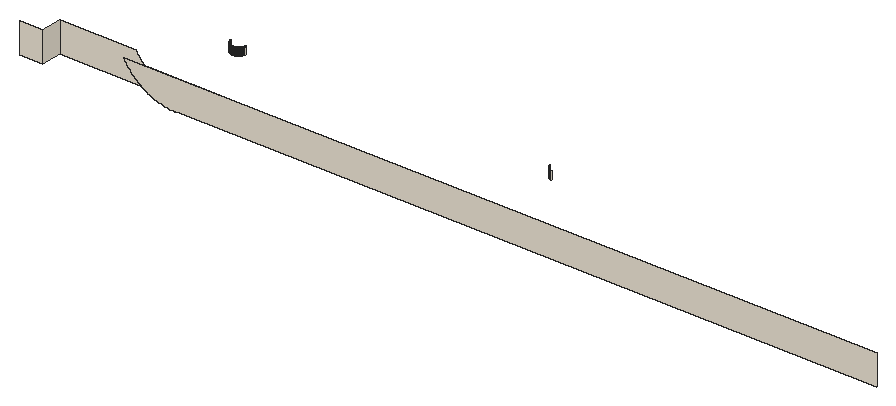
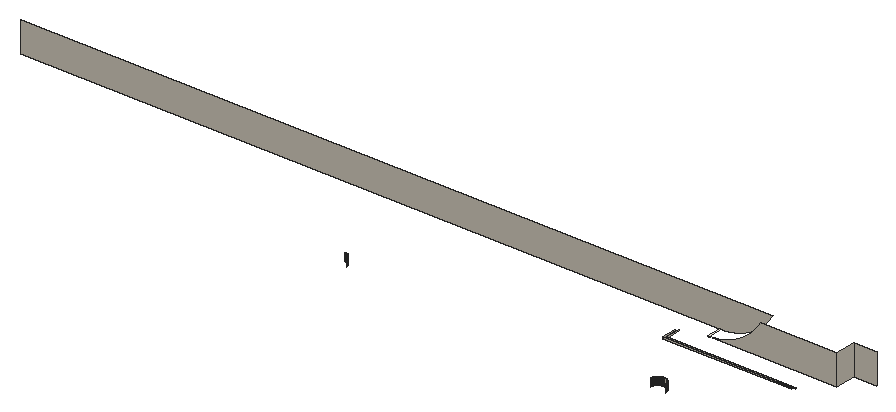
# SketchUp Ruby script. Lengths in inches.
U = 1.inch
M = Sketchup.active_model
def pt(a) = Geom::Point3d.new(a.map { |v| v * U })
def face(e, loops, mat)
  f = e.add_face(loops[0].map { |a| pt(a) })
  loops[1..].each { |l| e.add_face(l.map { |a| pt(a) }).erase! }
  f.material = f.back_material = mat if mat
  f
end
# faces: each face lists its corners as indices into pts; further lists are holes
def faces(e, pts, list, mat = nil) = list.each { |f| face(e, (f[0].is_a?(Array) ? f : [f]).map { |l| l.map { |i| pts[i] } }, mat) }
# xy, xz, yz: faces in a plane at the given z, y or x. An outline is a flat list of corners, or four numbers for a rectangle; further outlines are holes
def ring(l) = l.size == 4 ? [[l[0], l[1]], [l[2], l[1]], [l[2], l[3]], [l[0], l[3]]] : l.each_slice(2).to_a
def flat(e, list, mat, &to3) = list.each { |f| face(e, (f[0].is_a?(Array) ? f : [f]).map { |l| ring(l).map { |u, v| to3.(u, v) } }, mat) }
def xy(e, z, list, mat = nil) = flat(e, list, mat) { |x, y| [x, y, z] }
def xz(e, y, list, mat = nil) = flat(e, list, mat) { |x, z| [x, y, z] }
def yz(e, x, list, mat = nil) = flat(e, list, mat) { |y, z| [x, y, z] }
def lines(e, pts, list) = list.each { |a, b| e.add_line(pt(pts[a]), pt(pts[b])) }
# prism: a flat outline (further loops are holes) pulled along v
def prism(e, loops, v, mat = nil)
  f = face(e, loops, mat); d = Geom::Vector3d.new(v.map { |x| x * U })
  f.pushpull(f.normal.samedirection?(d) ? d.length : -d.length)
end
def box(e, o, s, mat = nil) = prism(e, [[o, [o[0] + s[0], o[1], o[2]], [o[0] + s[0], o[1] + s[1], o[2]], [o[0], o[1] + s[1], o[2]]]], [0, 0, s[2]], mat)
def at(x, y, z, deg = 0) = Geom::Transformation.translation(pt([x, y, z])) * Geom::Transformation.rotation(ORIGIN, Z_AXIS, deg.degrees)
def axes(o, x, y, z) = Geom::Transformation.new([*x, 0, *y, 0, *z, 0, *pt(o).to_a, 1])
def part(name) = M.definitions.add(name)
# library, detail: a bought-in or finely detailed component or shape, given as its bounding box
def library(name, o, s) = part(name).tap { |d| box(d.entities, o, s) }
def detail(e, o, s) = box(e.add_group.entities, o, s)
def put(e, d, t, mat = nil) = e.add_instance(d, t).tap { |i| i.material = mat if mat }
def group(e, t, mat = nil) = e.add_group.tap { |g| g.transformation = t; g.material = mat if mat }.entities
root = M.entities
M.materials.add("0027 AP L140 CRUSHED ICE").color = [241, 233, 217]
xz(root,214,[[9,120,18,132]],"0027 AP L140 CRUSHED ICE")
xz(root,216,[[69,120,345,120,345,132,48.22,132,48.47,131.57,48.74,131.14,49.01,130.72,49.29,130.3,49.58,129.89,49.88,129.49,50.19,129.09,50.51,128.7,50.83,128.32,51.16,127.94,51.51,127.57,51.85,127.21,52.21,126.85,52.57,126.5,52.94,126.16,53.32,125.83,53.7,125.51,54.09,125.19,54.49,124.88,54.89,124.58,55.3,124.29,55.72,124.01,56.14,123.74,56.57,123.47,57,123.22,57.4375,122.97,57.88,122.73,58.33,122.5,58.78,122.28,59.24,122.08,59.7,121.875,60.17,121.69,60.63,121.51,61.11,121.34,61.58,121.17,62.0625,121.02,62.55,120.88,63.03,120.75,63.52,120.63,64.01,120.52,64.5,120.43,65,120.34,65.49,120.26,65.99,120.1875,66.49,120.13,66.99,120.08,67.99,120.02,68.5,120.01]],"0027 AP L140 CRUSHED ICE")
xz(root,222,[[18,120,69,120,68.5,120.01,67.99,120.02,66.99,120.08,66.49,120.13,65.99,120.1875,65.49,120.26,65,120.34,64.5,120.43,64.01,120.52,63.52,120.63,63.03,120.75,62.55,120.88,62.0625,121.02,61.58,121.17,61.11,121.34,60.63,121.51,60.17,121.69,59.7,121.875,59.24,122.08,58.78,122.28,58.33,122.5,57.88,122.73,57.4375,122.97,57,123.22,56.57,123.47,56.14,123.74,55.72,124.01,55.3,124.29,54.89,124.58,54.49,124.88,54.09,125.19,53.7,125.51,53.32,125.83,52.94,126.16,52.57,126.5,52.21,126.85,51.85,127.21,51.51,127.57,51.16,127.94,50.83,128.32,50.51,128.7,50.19,129.09,49.88,129.49,49.58,129.89,49.29,130.3,49.01,130.72,48.74,131.14,48.47,131.57,48.22,132,18,132]],"0027 AP L140 CRUSHED ICE")
xz(root,231,[[27,120,78,120.5]],"0027 AP L140 CRUSHED ICE")
xz(root,232,[[28,120,79,120.5]],"0027 AP L140 CRUSHED ICE")
xz(root,255,[[59.84,120,59.92,123],[59.92,120,60,123],[60,120,60.08,123],[60.08,120,60.16,123]],"0027 AP L140 CRUSHED ICE")
yz(root,18,[[214,120,222,132]],"0027 AP L140 CRUSHED ICE")
yz(root,78,[[225,120,231,120.5]],"0027 AP L140 CRUSHED ICE")
yz(root,79,[[226,120,232,120.5]],"0027 AP L140 CRUSHED ICE")
p = [[69,216,120],[68.5,216,120.01],[68.5,222,120.01],[69,222,120],[59.53,255.04,120],[59.45,255.05,120],
  [59.45,255.05,123],[59.53,255.04,123],[59.61,255.03,120],[59.61,255.03,123],[59.6875,255.02,120],[59.6875,255.02,123],
  [59.76,255.01,120],[59.76,255.01,123],[59.84,255,120],[59.84,255,123],[60.24,255.01,120],[60.16,255,120],
  [60.16,255,123],[60.24,255.01,123],[60.3125,255.02,120],[60.3125,255.02,123],[60.39,255.03,120],[60.39,255.03,123],
  [60.47,255.04,120],[60.47,255.04,123],[60.55,255.05,120],[60.55,255.05,123],[185.53,255.04,120],[185.45,255.05,120],
  [185.45,255.05,123],[185.53,255.04,123],[185.61,255.03,120],[185.61,255.03,123],[59.07,255.15,120],[59,255.17,120],
  [59,255.17,123],[59.07,255.15,123],[59.15,255.125,120],[59.15,255.125,123],[59.22,255.1,120],[59.22,255.1,123],
  [59.3,255.08,120],[59.3,255.08,123],[59.375,255.07,120],[59.375,255.07,123],[60.625,255.07,120],[60.625,255.07,123],
  [60.7,255.08,120],[60.7,255.08,123],[60.78,255.1,120],[60.78,255.1,123],[60.85,255.125,120],[60.85,255.125,123],
  [60.93,255.15,120],[60.93,255.15,123],[61,255.17,120],[61,255.17,123],[185.07,255.15,120],[185,255.17,120],
  [185,255.17,123],[185.07,255.15,123],[185.15,255.125,120],[185.15,255.125,123],[185.22,255.1,120],[185.22,255.1,123],
  [185.3,255.08,120],[185.3,255.08,123],[185.375,255.07,120],[185.375,255.07,123],[58.85,255.23,120],[58.78,255.26,120],
  [58.78,255.26,123],[58.85,255.23,123],[58.92,255.2,120],[58.92,255.2,123],[61.08,255.2,120],[61.08,255.2,123],
  [61.15,255.23,120],[61.15,255.23,123],[61.22,255.26,120],[61.22,255.26,123],[184.85,255.23,120],[184.78,255.26,120],
  [184.78,255.26,123],[184.85,255.23,123],[184.92,255.2,120],[184.92,255.2,123],[58.64,255.33,120],[58.57,255.36,120],
  [58.57,255.36,123],[58.64,255.33,123],[58.71,255.29,120],[58.71,255.29,123],[61.29,255.29,120],[61.29,255.29,123],
  [61.36,255.33,120],[61.36,255.33,123],[61.43,255.36,120],[61.43,255.36,123],[184.64,255.33,120],[184.57,255.36,120],
  [184.57,255.36,123],[184.64,255.33,123],[184.71,255.29,120],[184.71,255.29,123],[58.43,255.44,120],[58.37,255.48,120],
  [58.37,255.48,123],[58.43,255.44,123],[58.5,255.4,120],[58.5,255.4,123],[61.5,255.4,120],[61.5,255.4,123],
  [61.57,255.44,120],[61.57,255.44,123],[61.63,255.48,120],[61.63,255.48,123],[184.43,255.44,120],[184.37,255.48,120],
  [184.37,255.48,123],[184.43,255.44,123],[184.5,255.4,120],[184.5,255.4,123],[58.3,255.53,120],[58.24,255.57,120],
  [58.24,255.57,123],[58.3,255.53,123],[61.7,255.53,120],[61.7,255.53,123],[61.76,255.57,120],[61.76,255.57,123],
  [184.3,255.53,120],[184.24,255.57,120],[184.24,255.57,123],[184.3,255.53,123],[58.17,255.62,120],[58.11,255.67,120],
  [58.11,255.67,123],[58.17,255.62,123],[61.83,255.62,120],[61.83,255.62,123],[61.89,255.67,120],[61.89,255.67,123],
  [184.17,255.62,120],[184.11,255.67,120],[184.11,255.67,123],[184.17,255.62,123],[58.05,255.72,120],[57.99,255.77,120],
  [57.99,255.77,123],[58.05,255.72,123],[61.95,255.72,120],[61.95,255.72,123],[62.01,255.77,120],[62.01,255.77,123],
  [184.05,255.72,120],[183.99,255.77,120],[183.99,255.77,123],[184.05,255.72,123],[57.93,255.82,120],[57.88,255.88,120],
  [57.88,255.88,123],[57.93,255.82,123],[62.07,255.82,120],[62.07,255.82,123],[62.12,255.88,120],[62.12,255.88,123],
  [183.93,255.82,120],[183.88,255.88,120],[183.88,255.88,123],[183.93,255.82,123],[57.82,255.93,120],[57.77,255.99,120],
  [57.77,255.99,123],[57.82,255.93,123],[62.18,255.93,120],[62.18,255.93,123],[62.23,255.99,120],[62.23,255.99,123],
  [183.82,255.93,120],[183.77,255.99,120],[183.77,255.99,123],[183.82,255.93,123],[57.72,256.05,120],[57.72,256.05,123],
  [62.28,256.05,120],[62.28,256.05,123],[183.72,256.05,120],[183.72,256.05,123],[57.67,256.11,120],[57.62,256.17,120],
  [57.62,256.17,123],[57.67,256.11,123],[62.33,256.11,120],[62.33,256.11,123],[62.38,256.17,120],[62.38,256.17,123],
  [183.67,256.11,120],[183.62,256.17,120],[183.62,256.17,123],[183.67,256.11,123],[57.57,256.24,120],[57.53,256.3,120],
  [57.53,256.3,123],[57.57,256.24,123],[62.43,256.24,120],[62.43,256.24,123],[62.47,256.3,120],[62.47,256.3,123],
  [183.57,256.24,120],[183.53,256.3,120],[183.53,256.3,123],[183.57,256.24,123],[57.48,256.37,120],[57.48,256.37,123],
  [62.52,256.37,120],[62.52,256.37,123],[183.48,256.37,120],[183.48,256.37,123],[57.44,256.43,120],[57.4,256.5,120],
  [57.4,256.5,123],[57.44,256.43,123],[62.56,256.43,120],[62.56,256.43,123],[62.6,256.5,120],[62.6,256.5,123],
  [183.44,256.43,120],[183.4,256.5,120],[183.4,256.5,123],[183.44,256.43,123],[57.36,256.57,120],[57.36,256.57,123],
  [62.64,256.57,120],[62.64,256.57,123],[183.36,256.57,120],[183.36,256.57,123],[57.33,256.64,120],[57.29,256.71,120],
  [57.29,256.71,123],[57.33,256.64,123],[62.67,256.64,120],[62.67,256.64,123],[62.71,256.71,120],[62.71,256.71,123],
  [183.33,256.64,120],[183.29,256.71,120],[183.29,256.71,123],[183.33,256.64,123],[57.26,256.78,120],[57.26,256.78,123],
  [62.74,256.78,120],[62.74,256.78,123],[183.26,256.78,120],[183.26,256.78,123],[57.23,256.85,120],[57.23,256.85,123],
  [62.77,256.85,120],[62.77,256.85,123],[183.23,256.85,120],[183.23,256.85,123],[57.2,256.92,120],[57.17,257,120],
  [57.17,257,123],[57.2,256.92,123],[62.8,256.92,120],[62.8,256.92,123],[62.83,257,120],[62.83,257,123],
  [183.2,256.92,120],[183.17,257,120],[183.17,257,123],[183.2,256.92,123],[57.15,257.07,120],[57.15,257.07,123],
  [62.85,257.07,120],[62.85,257.07,123],[183.15,257.07,120],[183.15,257.07,123],[57.125,257.15,120],[57.1,257.22,120],
  [57.1,257.22,123],[57.125,257.15,123],[62.875,257.15,120],[62.875,257.15,123],[62.9,257.22,120],[62.9,257.22,123],
  [183.125,257.15,120],[183.1,257.22,120],[183.1,257.22,123],[183.125,257.15,123],[57.08,257.3,120],[57.08,257.3,123],
  [62.92,257.3,120],[62.92,257.3,123],[183.08,257.3,120],[183.08,257.3,123],[57.07,257.375,120],[57.07,257.375,123],
  [62.93,257.375,120],[62.93,257.375,123],[183.07,257.375,120],[183.07,257.375,123],[57.05,257.45,120],[57.05,257.45,123],
  [62.95,257.45,120],[62.95,257.45,123],[183.05,257.45,120],[183.05,257.45,123],[57.04,257.53,120],[57.03,257.61,120],
  [57.03,257.61,123],[57.04,257.53,123],[62.96,257.53,120],[62.96,257.53,123],[62.97,257.61,120],[62.97,257.61,123],
  [183.04,257.53,120],[183.03,257.61,120],[183.03,257.61,123],[183.04,257.53,123],[57.02,257.6875,120],[57.02,257.6875,123],
  [183.02,257.6875,120],[183.02,257.6875,123]]
faces(root,p,[[0,1,2,3],[4,5,6,7],[8,4,7,9],[10,8,9,11],[12,10,11,13],[14,12,13,15],[16,17,18,19],[20,16,19,21],
  [22,20,21,23],[24,22,23,25],[26,24,25,27],[28,29,30,31],[32,28,31,33],[34,35,36,37],[38,34,37,39],[40,38,39,41],
  [42,40,41,43],[44,42,43,45],[5,44,45,6],[46,26,27,47],[48,46,47,49],[50,48,49,51],[52,50,51,53],[54,52,53,55],
  [56,54,55,57],[58,59,60,61],[62,58,61,63],[64,62,63,65],[66,64,65,67],[68,66,67,69],[29,68,69,30],[70,71,72,73],
  [74,70,73,75],[35,74,75,36],[76,56,57,77],[78,76,77,79],[80,78,79,81],[82,83,84,85],[86,82,85,87],[59,86,87,60],
  [88,89,90,91],[92,88,91,93],[71,92,93,72],[94,80,81,95],[96,94,95,97],[98,96,97,99],[100,101,102,103],[104,100,103,105],
  [83,104,105,84],[106,107,108,109],[110,106,109,111],[89,110,111,90],[112,98,99,113],[114,112,113,115],[116,114,115,117],[118,119,120,121],
  [122,118,121,123],[101,122,123,102],[124,125,126,127],[107,124,127,108],[128,116,117,129],[130,128,129,131],[132,133,134,135],[119,132,135,120],
  [136,137,138,139],[125,136,139,126],[140,130,131,141],[142,140,141,143],[144,145,146,147],[133,144,147,134],[148,149,150,151],[137,148,151,138],
  [152,142,143,153],[154,152,153,155],[156,157,158,159],[145,156,159,146],[160,161,162,163],[149,160,163,150],[164,154,155,165],[166,164,165,167],
  [168,169,170,171],[157,168,171,158],[172,173,174,175],[161,172,175,162],[176,166,167,177],[178,176,177,179],[180,181,182,183],[169,180,183,170],
  [173,184,185,174],[186,178,179,187],[181,188,189,182],[190,191,192,193],[184,190,193,185],[194,186,187,195],[196,194,195,197],[198,199,200,201],
  [188,198,201,189],[202,203,204,205],[191,202,205,192],[206,196,197,207],[208,206,207,209],[210,211,212,213],[199,210,213,200],[203,214,215,204],
  [216,208,209,217],[211,218,219,212],[220,221,222,223],[214,220,223,215],[224,216,217,225],[226,224,225,227],[228,229,230,231],[218,228,231,219],
  [221,232,233,222],[234,226,227,235],[229,236,237,230],[238,239,240,241],[232,238,241,233],[242,234,235,243],[244,242,243,245],[246,247,248,249],
  [236,246,249,237],[239,250,251,240],[252,244,245,253],[247,254,255,248],[250,256,257,251],[258,252,253,259],[254,260,261,255],[262,263,264,265],
  [256,262,265,257],[266,258,259,267],[268,266,267,269],[270,271,272,273],[260,270,273,261],[263,274,275,264],[276,268,269,277],[271,278,279,272],
  [280,281,282,283],[274,280,283,275],[284,276,277,285],[286,284,285,287],[288,289,290,291],[278,288,291,279],[281,292,293,282],[294,286,287,295],
  [289,296,297,290],[292,298,299,293],[300,294,295,301],[296,302,303,297],[298,304,305,299],[306,300,301,307],[302,308,309,303],[310,311,312,313],
  [304,310,313,305],[314,306,307,315],[316,314,315,317],[318,319,320,321],[308,318,321,309],[311,322,323,312],[319,324,325,320]],"0027 AP L140 CRUSHED ICE")
